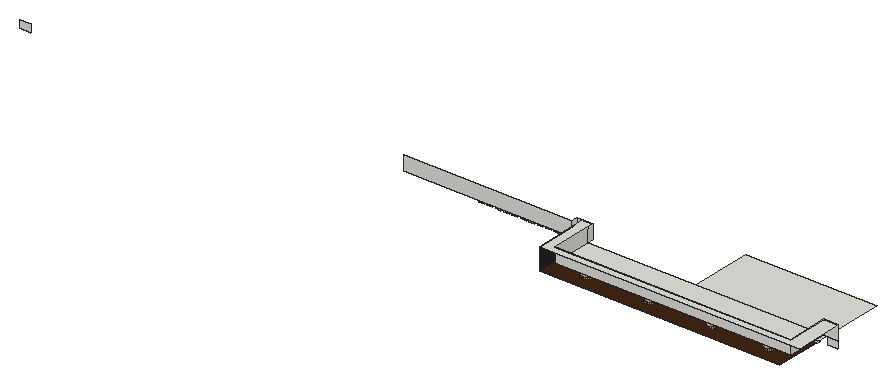
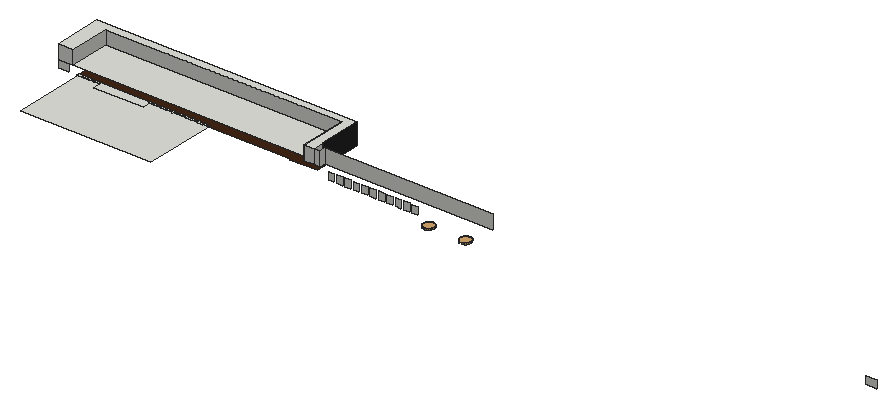
# SketchUp Ruby script. Lengths in inches.
U = 1.inch
M = Sketchup.active_model
def pt(a) = Geom::Point3d.new(a.map { |v| v * U })
def face(e, loops, mat)
  f = e.add_face(loops[0].map { |a| pt(a) })
  loops[1..].each { |l| e.add_face(l.map { |a| pt(a) }).erase! }
  f.material = f.back_material = mat if mat
  f
end
# faces: each face lists its corners as indices into pts; further lists are holes
def faces(e, pts, list, mat = nil) = list.each { |f| face(e, (f[0].is_a?(Array) ? f : [f]).map { |l| l.map { |i| pts[i] } }, mat) }
# xy, xz, yz: faces in a plane at the given z, y or x. An outline is a flat list of corners, or four numbers for a rectangle; further outlines are holes
def ring(l) = l.size == 4 ? [[l[0], l[1]], [l[2], l[1]], [l[2], l[3]], [l[0], l[3]]] : l.each_slice(2).to_a
def flat(e, list, mat, &to3) = list.each { |f| face(e, (f[0].is_a?(Array) ? f : [f]).map { |l| ring(l).map { |u, v| to3.(u, v) } }, mat) }
def xy(e, z, list, mat = nil) = flat(e, list, mat) { |x, y| [x, y, z] }
def xz(e, y, list, mat = nil) = flat(e, list, mat) { |x, z| [x, y, z] }
def yz(e, x, list, mat = nil) = flat(e, list, mat) { |y, z| [x, y, z] }
def lines(e, pts, list) = list.each { |a, b| e.add_line(pt(pts[a]), pt(pts[b])) }
# prism: a flat outline (further loops are holes) pulled along v
def prism(e, loops, v, mat = nil)
  f = face(e, loops, mat); d = Geom::Vector3d.new(v.map { |x| x * U })
  f.pushpull(f.normal.samedirection?(d) ? d.length : -d.length)
end
def box(e, o, s, mat = nil) = prism(e, [[o, [o[0] + s[0], o[1], o[2]], [o[0] + s[0], o[1] + s[1], o[2]], [o[0], o[1] + s[1], o[2]]]], [0, 0, s[2]], mat)
def at(x, y, z, deg = 0) = Geom::Transformation.translation(pt([x, y, z])) * Geom::Transformation.rotation(ORIGIN, Z_AXIS, deg.degrees)
def axes(o, x, y, z) = Geom::Transformation.new([*x, 0, *y, 0, *z, 0, *pt(o).to_a, 1])
def part(name) = M.definitions.add(name)
# library, detail: a bought-in or finely detailed component or shape, given as its bounding box
def library(name, o, s) = part(name).tap { |d| box(d.entities, o, s) }
def detail(e, o, s) = box(e.add_group.entities, o, s)
def put(e, d, t, mat = nil) = e.add_instance(d, t).tap { |i| i.material = mat if mat }
def group(e, t, mat = nil) = e.add_group.tap { |g| g.transformation = t; g.material = mat if mat }.entities
root = M.entities
M.materials.add("[Field Square Tile]").color = [211, 167, 108]
M.materials.add("[Granite Dark Gray]").color = [38, 37, 37]
M.materials.add("[Wood Veneer 01]").color = [66, 38, 20]
xy(root,380.5,[[3170.71,2343.96,3176.13,2346.71],[3176.13,2343.96,3177.33,2346.71],[3177.33,2343.96,3182.76,2346.71],[3182.76,2343.96,3183.96,2346.71],[3183.96,2343.96,3189.38,2346.71],
  [3189.38,2343.96,3190.58,2346.71],[3190.58,2343.96,3196.01,2346.71],[3196.01,2343.96,3197.21,2346.71],[3197.21,2343.96,3202.63,2346.71],[3202.63,2343.96,3203.83,2346.71],
  [3203.83,2343.96,3209.26,2346.71],[3209.26,2343.96,3210.46,2346.71],[3210.46,2343.96,3215.88,2346.71],[3215.88,2343.96,3217.08,2346.71],[3217.08,2343.96,3222.51,2346.71],
  [3222.51,2343.96,3223.71,2346.71],[3223.71,2343.96,3229.13,2346.71],[3229.13,2343.96,3230.33,2346.71],[3230.33,2343.96,3235.76,2346.71],[3235.76,2343.96,3289.31,2354.27],
  [3289.31,2343.96,3294.73,2346.71],[3294.73,2343.96,3295.93,2346.71],[3295.93,2343.96,3301.36,2346.71],[3301.36,2343.96,3302.56,2346.71],[3302.56,2343.96,3307.98,2346.71],
  [3307.98,2343.96,3308.81,2346.71],[3308.81,2343.96,3312.79,2346.71],[3312.79,2343.96,3314.23,2346.71],[3170.71,2346.71,3170.71,2425.46,3312.79,2425.46,3312.79,2346.71,3289.31,2346.71,3289.31,2354.27,3235.76,2354.27,3235.76,2346.71]])
xy(root,380.5,[[[3051.23,2294.125,3051.23,2347.9,3081.03,2347.9,3081.03,2346.71,3170.71,2346.71,3170.71,2343.96,3312.79,2343.96,3312.79,2294.125],[3286.58,2306.32,3288.14,2306.53,3289.58,2307.13,3290.83,2308.08,3291.78,2309.32,3292.38,2310.77,3292.58,2312.32,3292.38,2313.88,3291.78,2315.32,3290.83,2316.57,3289.58,2317.52,3288.14,2318.12,3286.58,2318.32,3285.03,2318.12,3283.58,2317.52,3282.34,2316.57,3281.39,2315.32,3280.79,2313.88,3280.58,2312.32,3280.79,2310.77,3281.39,2309.32,3282.34,2308.08,3283.58,2307.13,3285.03,2306.53],[3088.47,2306.32,3090.02,2306.53,3091.47,2307.13,3092.71,2308.08,3093.66,2309.32,3094.26,2310.77,3094.47,2312.32,3094.26,2313.88,3093.66,2315.32,3092.71,2316.57,3091.47,2317.52,3090.02,2318.12,3088.47,2318.32,3086.92,2318.12,3085.47,2317.52,3084.23,2316.57,3083.27,2315.32,3082.67,2313.88,3082.47,2312.32,3082.67,2310.77,3083.27,2309.32,3084.23,2308.08,3085.47,2307.13,3086.92,2306.53],[3157.93,2306.32,3159.48,2306.53,3160.93,2307.13,3162.17,2308.08,3163.13,2309.32,3163.73,2310.77,3163.93,2312.32,3163.73,2313.88,3163.13,2315.32,3162.17,2316.57,3160.93,2317.52,3159.48,2318.12,3157.93,2318.32,3156.38,2318.12,3154.93,2317.52,3153.6875,2316.57,3152.74,2315.32,3152.14,2313.88,3151.93,2312.32,3152.14,2310.77,3152.74,2309.32,3153.6875,2308.08,3154.93,2307.13,3156.38,2306.53],[3225.21,2306.32,3226.76,2306.53,3228.21,2307.13,3229.45,2308.08,3230.41,2309.32,3231.01,2310.77,3231.21,2312.32,3231.01,2313.88,3230.41,2315.32,3229.45,2316.57,3228.21,2317.52,3226.76,2318.12,3225.21,2318.32,3223.66,2318.12,3222.21,2317.52,3220.97,2316.57,3220.01,2315.32,3219.41,2313.88,3219.21,2312.32,3219.41,2310.77,3220.01,2309.32,3220.97,2308.08,3222.21,2307.13,3223.66,2306.53]]],"[Wood Veneer 01]")
xy(root,381.8125,[[3088.47,2306.32,3086.92,2306.53,3085.47,2307.13,3084.23,2308.08,3083.27,2309.32,3082.67,2310.77,3082.47,2312.32,3082.67,2313.88,3083.27,2315.32,3084.23,2316.57,3085.47,2317.52,3086.92,2318.12,3088.47,2318.32,3090.02,2318.12,3091.47,2317.52,3092.71,2316.57,3093.66,2315.32,3094.26,2313.88,3094.47,2312.32,3094.26,2310.77,3093.66,2309.32,3092.71,2308.08,3091.47,2307.13,3090.02,2306.53],[3157.93,2306.32,3156.38,2306.53,3154.93,2307.13,3153.6875,2308.08,3152.74,2309.32,3152.14,2310.77,3151.93,2312.32,3152.14,2313.88,3152.74,2315.32,3153.6875,2316.57,3154.93,2317.52,3156.38,2318.12,3157.93,2318.32,3159.48,2318.12,3160.93,2317.52,3162.17,2316.57,3163.13,2315.32,3163.73,2313.88,3163.93,2312.32,3163.73,2310.77,3163.13,2309.32,3162.17,2308.08,3160.93,2307.13,3159.48,2306.53],[3225.21,2306.32,3223.66,2306.53,3222.21,2307.13,3220.97,2308.08,3220.01,2309.32,3219.41,2310.77,3219.21,2312.32,3219.41,2313.88,3220.01,2315.32,3220.97,2316.57,3222.21,2317.52,3223.66,2318.12,3225.21,2318.32,3226.76,2318.12,3228.21,2317.52,3229.45,2316.57,3230.41,2315.32,3231.01,2313.88,3231.21,2312.32,3231.01,2310.77,3230.41,2309.32,3229.45,2308.08,3228.21,2307.13,3226.76,2306.53],[3286.58,2306.32,3285.03,2306.53,3283.58,2307.13,3282.34,2308.08,3281.39,2309.32,3280.79,2310.77,3280.58,2312.32,3280.79,2313.88,3281.39,2315.32,3282.34,2316.57,3283.58,2317.52,3285.03,2318.12,3286.58,2318.32,3288.14,2318.12,3289.58,2317.52,3290.83,2316.57,3291.78,2315.32,3292.38,2313.88,3292.58,2312.32,3292.38,2310.77,3291.78,2309.32,3290.83,2308.08,3289.58,2307.13,3288.14,2306.53]],"[Field Square Tile]")
xy(root,381.875,[[2877.08,2359.13,2875.52,2359.16,2874.01,2359.6,2872.67,2360.41,2871.59,2361.54,2870.83,2362.91,2870.46,2364.4375,2870.49,2366,2870.93,2367.51,2871.74,2368.85,2872.87,2369.93,2874.24,2370.69,2875.76,2371.06,2877.33,2371.03,2878.83,2370.59,2880.17,2369.78,2881.26,2368.65,2882.01,2367.28,2882.39,2365.75,2882.35,2364.1875,2881.92,2362.68,2881.11,2361.34,2879.98,2360.26,2878.6,2359.51],[2916.83,2359.13,2915.27,2359.16,2913.76,2359.6,2912.42,2360.41,2911.34,2361.54,2910.58,2362.91,2910.21,2364.4375,2910.24,2366,2910.68,2367.51,2911.49,2368.85,2912.62,2369.93,2913.99,2370.69,2915.51,2371.06,2917.08,2371.03,2918.58,2370.59,2919.92,2369.78,2921.01,2368.65,2921.76,2367.28,2922.14,2365.75,2922.1,2364.1875,2921.67,2362.68,2920.86,2361.34,2919.73,2360.26,2918.35,2359.51]],"[Field Square Tile]")
xy(root,388.625,[[3061.9375,2301.68,3318.43,2346.71]])
xy(root,403.8125,[[3051.23,2294.125,3334.41,2294.125,3334.41,2346.71,3318.43,2346.71,3318.43,2301.68,3061.9375,2301.68,3061.9375,2353.05,3051.23,2353.05]])
xz(root,2301.68,[[3061.9375,388.625,3318.43,403.8125]])
xz(root,2346.49,[[2861.56,388.625,3044.88,403.8125]])
xz(root,2346.71,[[2443.85,380.5,2455.66,388.625],[3322.6,380.5,3334.41,388.625],[3318.43,388.625,3334.41,403.8125]])
xz(root,2353.05,[[3044.88,388.625,3051.23,403.8125],[3051.23,388.625,3061.9375,403.8125]])
xz(root,2355.06,[[2936.18,380.5,2942.43,388.625],[2945.31,380.5,2951.56,388.625],[2954.43,380.5,2960.68,388.625],[2963.56,380.5,2969.81,388.625],[2972.68,380.5,2978.93,388.625],
  [2981.81,380.5,2988.06,388.625],[2990.93,380.5,2997.18,388.625],[3000.06,380.5,3006.31,388.625],[3009.18,380.5,3015.43,388.625],[3018.31,380.5,3024.56,388.625],
  [3027.43,380.5,3033.68,388.625]])
yz(root,3044.88,[[2346.49,388.625,2353.05,403.8125]])
yz(root,3051.23,[[2294.125,380.5,2340.15,403.8125]],"[Granite Dark Gray]")
yz(root,3061.9375,[[2301.68,388.625,2346.71,403.8125],[2346.71,388.625,2353.05,403.8125]])
yz(root,3318.43,[[2301.68,388.625,2346.71,403.8125]])
p = [[3088.47,2306.32,380.5],[3086.92,2306.53,380.5],[3086.92,2306.53,381.8125],[3088.47,2306.32,381.8125],[3090.02,2306.53,380.5],[3090.02,2306.53,381.8125],
  [3157.93,2306.32,380.5],[3156.38,2306.53,380.5],[3156.38,2306.53,381.8125],[3157.93,2306.32,381.8125],[3159.48,2306.53,380.5],[3159.48,2306.53,381.8125],
  [3225.21,2306.32,380.5],[3223.66,2306.53,380.5],[3223.66,2306.53,381.8125],[3225.21,2306.32,381.8125],[3226.76,2306.53,380.5],[3226.76,2306.53,381.8125],
  [3286.58,2306.32,380.5],[3285.03,2306.53,380.5],[3285.03,2306.53,381.8125],[3286.58,2306.32,381.8125],[3288.14,2306.53,380.5],[3288.14,2306.53,381.8125],
  [3085.47,2307.13,380.5],[3085.47,2307.13,381.8125],[3091.47,2307.13,380.5],[3091.47,2307.13,381.8125],[3154.93,2307.13,380.5],[3154.93,2307.13,381.8125],
  [3160.93,2307.13,380.5],[3160.93,2307.13,381.8125],[3222.21,2307.13,380.5],[3222.21,2307.13,381.8125],[3228.21,2307.13,380.5],[3228.21,2307.13,381.8125],
  [3283.58,2307.13,380.5],[3283.58,2307.13,381.8125],[3289.58,2307.13,380.5],[3289.58,2307.13,381.8125],[3084.23,2308.08,380.5],[3084.23,2308.08,381.8125],
  [3092.71,2308.08,380.5],[3092.71,2308.08,381.8125],[3153.6875,2308.08,380.5],[3153.6875,2308.08,381.8125],[3162.17,2308.08,380.5],[3162.17,2308.08,381.8125],
  [3220.97,2308.08,380.5],[3220.97,2308.08,381.8125],[3229.45,2308.08,380.5],[3229.45,2308.08,381.8125],[3282.34,2308.08,380.5],[3282.34,2308.08,381.8125],
  [3290.83,2308.08,380.5],[3290.83,2308.08,381.8125],[3083.27,2309.32,380.5],[3083.27,2309.32,381.8125],[3093.66,2309.32,380.5],[3093.66,2309.32,381.8125],
  [3152.74,2309.32,380.5],[3152.74,2309.32,381.8125],[3163.13,2309.32,380.5],[3163.13,2309.32,381.8125],[3220.01,2309.32,380.5],[3220.01,2309.32,381.8125],
  [3230.41,2309.32,380.5],[3230.41,2309.32,381.8125],[3281.39,2309.32,380.5],[3281.39,2309.32,381.8125],[3291.78,2309.32,380.5],[3291.78,2309.32,381.8125],
  [3082.67,2310.77,380.5],[3082.67,2310.77,381.8125],[3094.26,2310.77,380.5],[3094.26,2310.77,381.8125],[3152.14,2310.77,380.5],[3152.14,2310.77,381.8125],
  [3163.73,2310.77,380.5],[3163.73,2310.77,381.8125],[3219.41,2310.77,380.5],[3219.41,2310.77,381.8125],[3231.01,2310.77,380.5],[3231.01,2310.77,381.8125],
  [3280.79,2310.77,380.5],[3280.79,2310.77,381.8125],[3292.38,2310.77,380.5],[3292.38,2310.77,381.8125],[3082.47,2312.32,380.5],[3082.47,2312.32,381.8125],
  [3094.47,2312.32,380.5],[3094.47,2312.32,381.8125],[3151.93,2312.32,380.5],[3151.93,2312.32,381.8125],[3163.93,2312.32,380.5],[3163.93,2312.32,381.8125],
  [3219.21,2312.32,380.5],[3219.21,2312.32,381.8125],[3231.21,2312.32,380.5],[3231.21,2312.32,381.8125],[3280.58,2312.32,380.5],[3280.58,2312.32,381.8125],
  [3292.58,2312.32,380.5],[3292.58,2312.32,381.8125],[3082.67,2313.88,380.5],[3082.67,2313.88,381.8125],[3094.26,2313.88,380.5],[3094.26,2313.88,381.8125],
  [3152.14,2313.88,380.5],[3152.14,2313.88,381.8125],[3163.73,2313.88,380.5],[3163.73,2313.88,381.8125],[3219.41,2313.88,380.5],[3219.41,2313.88,381.8125],
  [3231.01,2313.88,380.5],[3231.01,2313.88,381.8125],[3280.79,2313.88,380.5],[3280.79,2313.88,381.8125],[3292.38,2313.88,380.5],[3292.38,2313.88,381.8125],
  [3083.27,2315.32,380.5],[3083.27,2315.32,381.8125],[3093.66,2315.32,380.5],[3093.66,2315.32,381.8125],[3152.74,2315.32,380.5],[3152.74,2315.32,381.8125],
  [3163.13,2315.32,380.5],[3163.13,2315.32,381.8125],[3220.01,2315.32,380.5],[3220.01,2315.32,381.8125],[3230.41,2315.32,380.5],[3230.41,2315.32,381.8125],
  [3281.39,2315.32,380.5],[3281.39,2315.32,381.8125],[3291.78,2315.32,380.5],[3291.78,2315.32,381.8125],[3084.23,2316.57,380.5],[3084.23,2316.57,381.8125],
  [3092.71,2316.57,380.5],[3092.71,2316.57,381.8125],[3153.6875,2316.57,380.5],[3153.6875,2316.57,381.8125],[3162.17,2316.57,380.5],[3162.17,2316.57,381.8125],
  [3220.97,2316.57,380.5],[3220.97,2316.57,381.8125],[3229.45,2316.57,380.5],[3229.45,2316.57,381.8125],[3282.34,2316.57,380.5],[3282.34,2316.57,381.8125],
  [3290.83,2316.57,380.5],[3290.83,2316.57,381.8125],[3085.47,2317.52,380.5],[3085.47,2317.52,381.8125],[3091.47,2317.52,380.5],[3091.47,2317.52,381.8125],
  [3154.93,2317.52,380.5],[3154.93,2317.52,381.8125],[3160.93,2317.52,380.5],[3160.93,2317.52,381.8125],[3222.21,2317.52,380.5],[3222.21,2317.52,381.8125],
  [3228.21,2317.52,380.5],[3228.21,2317.52,381.8125],[3283.58,2317.52,380.5],[3283.58,2317.52,381.8125],[3289.58,2317.52,380.5],[3289.58,2317.52,381.8125],
  [3086.92,2318.12,380.5],[3086.92,2318.12,381.8125],[3090.02,2318.12,380.5],[3090.02,2318.12,381.8125],[3156.38,2318.12,380.5],[3156.38,2318.12,381.8125],
  [3159.48,2318.12,380.5],[3159.48,2318.12,381.8125],[3223.66,2318.12,380.5],[3223.66,2318.12,381.8125],[3226.76,2318.12,380.5],[3226.76,2318.12,381.8125],
  [3285.03,2318.12,380.5],[3285.03,2318.12,381.8125],[3288.14,2318.12,380.5],[3288.14,2318.12,381.8125],[3088.47,2318.32,380.5],[3088.47,2318.32,381.8125],
  [3157.93,2318.32,380.5],[3157.93,2318.32,381.8125],[3225.21,2318.32,380.5],[3225.21,2318.32,381.8125],[3286.58,2318.32,380.5],[3286.58,2318.32,381.8125],
  [2877.08,2359.13,380.5],[2875.52,2359.16,380.5],[2875.52,2359.16,381.875],[2877.08,2359.13,381.875],[2878.6,2359.51,380.5],[2878.6,2359.51,381.875],
  [2916.83,2359.13,380.5],[2915.27,2359.16,380.5],[2915.27,2359.16,381.875],[2916.83,2359.13,381.875],[2918.35,2359.51,380.5],[2918.35,2359.51,381.875],
  [2874.01,2359.6,380.5],[2874.01,2359.6,381.875],[2913.76,2359.6,380.5],[2913.76,2359.6,381.875],[2879.98,2360.26,380.5],[2879.98,2360.26,381.875],
  [2919.73,2360.26,380.5],[2919.73,2360.26,381.875],[2872.67,2360.41,380.5],[2872.67,2360.41,381.875],[2912.42,2360.41,380.5],[2912.42,2360.41,381.875],
  [2881.11,2361.34,380.5],[2881.11,2361.34,381.875],[2920.86,2361.34,380.5],[2920.86,2361.34,381.875],[2871.59,2361.54,380.5],[2871.59,2361.54,381.875],
  [2911.34,2361.54,380.5],[2911.34,2361.54,381.875],[2881.92,2362.68,380.5],[2881.92,2362.68,381.875],[2921.67,2362.68,380.5],[2921.67,2362.68,381.875],
  [2870.83,2362.91,380.5],[2870.83,2362.91,381.875],[2910.58,2362.91,380.5],[2910.58,2362.91,381.875],[2882.35,2364.1875,380.5],[2882.35,2364.1875,381.875],
  [2922.1,2364.1875,380.5],[2922.1,2364.1875,381.875],[2870.46,2364.4375,380.5],[2870.46,2364.4375,381.875],[2910.21,2364.4375,380.5],[2910.21,2364.4375,381.875],
  [2882.39,2365.75,380.5],[2882.39,2365.75,381.875],[2922.14,2365.75,380.5],[2922.14,2365.75,381.875],[2870.49,2366,380.5],[2870.49,2366,381.875],
  [2910.24,2366,380.5],[2910.24,2366,381.875],[2882.01,2367.28,380.5],[2882.01,2367.28,381.875],[2921.76,2367.28,380.5],[2921.76,2367.28,381.875],
  [2870.93,2367.51,380.5],[2870.93,2367.51,381.875],[2910.68,2367.51,380.5],[2910.68,2367.51,381.875],[2881.26,2368.65,380.5],[2881.26,2368.65,381.875],
  [2921.01,2368.65,380.5],[2921.01,2368.65,381.875],[2871.74,2368.85,380.5],[2871.74,2368.85,381.875],[2911.49,2368.85,380.5],[2911.49,2368.85,381.875],
  [2880.17,2369.78,380.5],[2880.17,2369.78,381.875],[2919.92,2369.78,380.5],[2919.92,2369.78,381.875],[2872.87,2369.93,380.5],[2872.87,2369.93,381.875],
  [2912.62,2369.93,380.5],[2912.62,2369.93,381.875],[2878.83,2370.59,380.5],[2878.83,2370.59,381.875],[2918.58,2370.59,380.5],[2918.58,2370.59,381.875],
  [2874.24,2370.69,380.5],[2874.24,2370.69,381.875],[2913.99,2370.69,380.5],[2913.99,2370.69,381.875],[2877.33,2371.03,380.5],[2877.33,2371.03,381.875],
  [2917.08,2371.03,380.5],[2917.08,2371.03,381.875],[2875.76,2371.06,380.5],[2875.76,2371.06,381.875],[2915.51,2371.06,380.5],[2915.51,2371.06,381.875],
  [3051.25,2303.93,380.5],[3051.23,2294.125,380.5]]
faces(root,p,[[0,1,2,3],[4,0,3,5],[6,7,8,9],[10,6,9,11],[12,13,14,15],[16,12,15,17],[18,19,20,21],[22,18,21,23],
  [1,24,25,2],[26,4,5,27],[7,28,29,8],[30,10,11,31],[13,32,33,14],[34,16,17,35],[19,36,37,20],[38,22,23,39],
  [24,40,41,25],[42,26,27,43],[28,44,45,29],[46,30,31,47],[32,48,49,33],[50,34,35,51],[36,52,53,37],[54,38,39,55],
  [40,56,57,41],[58,42,43,59],[44,60,61,45],[62,46,47,63],[48,64,65,49],[66,50,51,67],[52,68,69,53],[70,54,55,71],
  [56,72,73,57],[74,58,59,75],[60,76,77,61],[78,62,63,79],[64,80,81,65],[82,66,67,83],[68,84,85,69],[86,70,71,87],
  [72,88,89,73],[90,74,75,91],[76,92,93,77],[94,78,79,95],[80,96,97,81],[98,82,83,99],[84,100,101,85],[102,86,87,103],
  [88,104,105,89],[106,90,91,107],[92,108,109,93],[110,94,95,111],[96,112,113,97],[114,98,99,115],[100,116,117,101],[118,102,103,119],
  [104,120,121,105],[122,106,107,123],[108,124,125,109],[126,110,111,127],[112,128,129,113],[130,114,115,131],[116,132,133,117],[134,118,119,135],
  [120,136,137,121],[138,122,123,139],[124,140,141,125],[142,126,127,143],[128,144,145,129],[146,130,131,147],[132,148,149,133],[150,134,135,151],
  [136,152,153,137],[154,138,139,155],[140,156,157,141],[158,142,143,159],[144,160,161,145],[162,146,147,163],[148,164,165,149],[166,150,151,167],
  [152,168,169,153],[170,154,155,171],[156,172,173,157],[174,158,159,175],[160,176,177,161],[178,162,163,179],[164,180,181,165],[182,166,167,183],
  [168,184,185,169],[184,170,171,185],[172,186,187,173],[186,174,175,187],[176,188,189,177],[188,178,179,189],[180,190,191,181],[190,182,183,191],
  [192,193,194,195],[196,192,195,197],[198,199,200,201],[202,198,201,203],[193,204,205,194],[199,206,207,200],[208,196,197,209],[210,202,203,211],
  [204,212,213,205],[206,214,215,207],[216,208,209,217],[218,210,211,219],[212,220,221,213],[214,222,223,215],[224,216,217,225],[226,218,219,227],
  [220,228,229,221],[222,230,231,223],[232,224,225,233],[234,226,227,235],[228,236,237,229],[230,238,239,231],[240,232,233,241],[242,234,235,243],
  [236,244,245,237],[238,246,247,239],[248,240,241,249],[250,242,243,251],[244,252,253,245],[246,254,255,247],[256,248,249,257],[258,250,251,259],
  [252,260,261,253],[254,262,263,255],[264,256,257,265],[266,258,259,267],[260,268,269,261],[262,270,271,263],[272,264,265,273],[274,266,267,275],
  [268,276,277,269],[270,278,279,271],[280,272,273,281],[282,274,275,283],[276,284,285,277],[278,286,287,279]],"[Field Square Tile]")
lines(root,p,[[288,289]])
